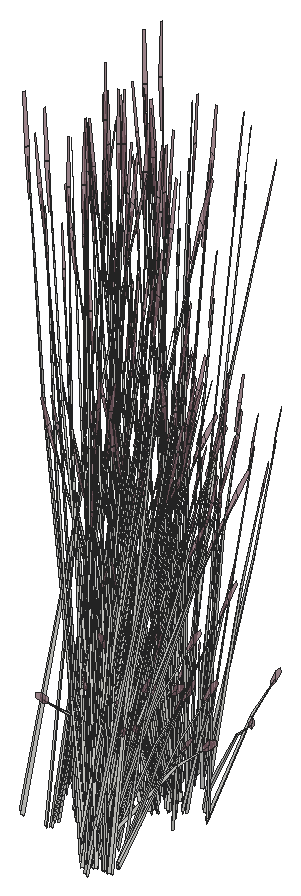
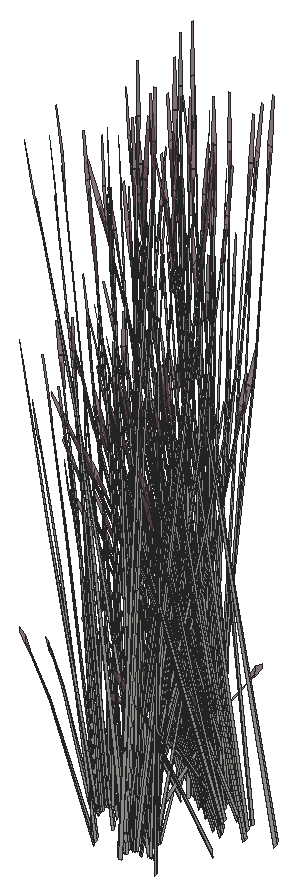
# SketchUp Ruby script. Lengths in inches.
U = 1.inch
M = Sketchup.active_model
def pt(a) = Geom::Point3d.new(a.map { |v| v * U })
def face(e, loops, mat)
  f = e.add_face(loops[0].map { |a| pt(a) })
  loops[1..].each { |l| e.add_face(l.map { |a| pt(a) }).erase! }
  f.material = f.back_material = mat if mat
  f
end
# faces: each face lists its corners as indices into pts; further lists are holes
def faces(e, pts, list, mat = nil) = list.each { |f| face(e, (f[0].is_a?(Array) ? f : [f]).map { |l| l.map { |i| pts[i] } }, mat) }
# xy, xz, yz: faces in a plane at the given z, y or x. An outline is a flat list of corners, or four numbers for a rectangle; further outlines are holes
def ring(l) = l.size == 4 ? [[l[0], l[1]], [l[2], l[1]], [l[2], l[3]], [l[0], l[3]]] : l.each_slice(2).to_a
def flat(e, list, mat, &to3) = list.each { |f| face(e, (f[0].is_a?(Array) ? f : [f]).map { |l| ring(l).map { |u, v| to3.(u, v) } }, mat) }
def xy(e, z, list, mat = nil) = flat(e, list, mat) { |x, y| [x, y, z] }
def xz(e, y, list, mat = nil) = flat(e, list, mat) { |x, z| [x, y, z] }
def yz(e, x, list, mat = nil) = flat(e, list, mat) { |y, z| [x, y, z] }
def lines(e, pts, list) = list.each { |a, b| e.add_line(pt(pts[a]), pt(pts[b])) }
# prism: a flat outline (further loops are holes) pulled along v
def prism(e, loops, v, mat = nil)
  f = face(e, loops, mat); d = Geom::Vector3d.new(v.map { |x| x * U })
  f.pushpull(f.normal.samedirection?(d) ? d.length : -d.length)
end
def box(e, o, s, mat = nil) = prism(e, [[o, [o[0] + s[0], o[1], o[2]], [o[0] + s[0], o[1] + s[1], o[2]], [o[0], o[1] + s[1], o[2]]]], [0, 0, s[2]], mat)
def at(x, y, z, deg = 0) = Geom::Transformation.translation(pt([x, y, z])) * Geom::Transformation.rotation(ORIGIN, Z_AXIS, deg.degrees)
def axes(o, x, y, z) = Geom::Transformation.new([*x, 0, *y, 0, *z, 0, *pt(o).to_a, 1])
def part(name) = M.definitions.add(name)
# library, detail: a bought-in or finely detailed component or shape, given as its bounding box
def library(name, o, s) = part(name).tap { |d| box(d.entities, o, s) }
def detail(e, o, s) = box(e.add_group.entities, o, s)
def put(e, d, t, mat = nil) = e.add_instance(d, t).tap { |i| i.material = mat if mat }
def group(e, t, mat = nil) = e.add_group.tap { |g| g.transformation = t; g.material = mat if mat }.entities
root = M.entities
M.materials.add("LightPink_Translucent").color = [144, 107, 117]
M.materials["LightPink_Translucent"].alpha = 0.75
c1 = part("blade")
p = [[2.15,0.21,22],[0,0.17,0],[0.09,0.45,0],[2.18,0.31,22],[2.29,0.31,22],[0.38,0.45,0],
  [2.48,0.24,33],[2.49,0.24,33],[2.48,0.22,33]]
faces(c1.entities,p,[[0,1,2,3],[4,5,2,3],[6,3,4,7],[8,0,3,6]])
c2 = part("seeds")
p = [[0.3,-0.1,1.38],[-0.01,-0.03,1.59],[-0.01,-0.03,0.03],[0.14,-0.07,-0.07],[0.29,-0.03,3],[0.15,0.01,3.11]]
faces(c2.entities,p,[[0,1,2,3],[1,0,4,5]],"LightPink_Translucent")
c3 = part("blade with seeds")
put(c3.entities,c1,at(0,0,0))
put(c3.entities,c2,axes([2.4,0.25,30.99],[1.5799,-0.05474,1.17369],[-0.12525,1.92788,0.29478],[-0.07173,-0.02425,1.56792]))
put(root,c3,axes([411.76,30.21,-9.7],[-0.40181,-0.39593,0.16428],[0.40492,-0.38402,0.32672],[-0.04438,0.08086,1.49371]))
put(root,c3,axes([411.01,29.61,-10.08],[0.53199,0.08911,-0.58063],[-0.11226,0.54969,-0.15239],[0.15876,0.06661,1.28164]))
put(root,c3,axes([413.37,30.57,-9.42],[-0.31598,0.08973,1.06958],[0.14873,-0.37085,0.78586],[0.16763,0.02538,0.23558]))
put(root,c3,axes([409.99,31.64,-9.95],[-0.51557,-0.24403,0],[0.24813,-0.50705,0],[0,0,1.51513]))
put(root,c3,axes([410.41,31,-9.7],[-0.49938,-0.43748,-0.23459],[0.42021,-0.49126,0.51337],[-0.13447,0.05118,1.56642]))
put(root,c3,axes([409.1,31.83,-9.69],[0.47863,0.27177,0.46235],[-0.28609,0.48733,0],[-0.10901,-0.0619,1.46668]))
put(root,c3,axes([405.94,33.55,-9.59],[-0.1827,-0.0161,1.33163],[-0.18717,-0.43188,-0.28638],[0.22444,-0.12218,0.56934]))
put(root,c3,axes([406.94,33.97,-7.62],[-0.0668,-0.00413,1.65179],[-0.27738,-0.44233,-0.15608],[0.11139,-0.14544,0.29231]))
put(root,c3,axes([410.79,29.95,-9.47],[0.24813,-0.48978,0.41661],[0.51557,0.23571,-0.2005],[0,0.1129,1.33761]))
put(root,c3,axes([413.22,32.14,-7.62],[-0.04624,-0.04758,1.65179],[0.10116,-0.51007,-0.15608],[0.18215,-0.03259,0.29231]))
put(root,c3,axes([406.15,32.76,-9.42],[-0.17034,0.27669,1.06958],[-0.14642,-0.37174,0.78586],[0.14069,-0.09315,0.23558]))
put(root,c3,axes([410.69,30.23,-9.87],[0,0.62861,-0.05249],[-0.63949,0,0],[0,0.01975,1.67027]))
put(root,c3,axes([410.74,29.79,-9.94],[0.30722,0.45622,-0.41661],[-0.46535,0.32126,0.2005],[0.09942,0.05645,1.33761]))
put(root,c3,axes([412.82,31.72,-8.34],[-0.09788,-0.45691,-0.03251],[0.46264,-0.10504,-0.14742],[0.09661,0.02897,0.48626]))
put(root,c3,axes([411.62,31.7,-7.3125],[0.02738,-0.55277,-0.11324],[0.51847,0.01511,-0.62851],[0.19968,0.0384,0.95501]))
put(root,c3,axes([405.91,33.8,-7.78],[0.44516,-0.07768,-0.32977],[0.11755,0.44407,0.42575],[0.12757,-0.11927,0.81462]))
put(root,c3,axes([412.09,30.23,-9.69],[0,-0.54355,0.46235],[0.57217,0,0],[0,0.1238,1.46668]))
put(root,c3,axes([410.66,30.63,-9.47],[0.55535,-0.03355,0.41661],[0.05022,0.55698,-0.2005],[-0.09942,0.05645,1.33761]))
put(root,c3,axes([411,30.06,-9.5625],[0.47648,-0.15851,0.13483],[0.16686,0.45265,-0.38503],[0,0.09962,1.18024]))
put(root,c3,axes([411.54,31.49,-7.3],[-0.29098,-0.34031,0.32977],[0.33226,-0.32215,-0.42575],[0.16881,0.04902,0.81462]))
put(root,c3,axes([410.16,30.9,-9.94],[-0.55535,0.03355,-0.41661],[-0.05022,-0.55698,0.2005],[-0.09942,0.05645,1.33761]))
put(root,c3,axes([412.77,31.17,-9.59],[-0.12317,-0.13368,1.33163],[0.16025,-0.44223,-0.28638],[0.24919,0.05991,0.56934]))
put(root,c3,axes([410.57,31.65,-9.95],[0.51557,0.24403,0],[-0.24813,0.50705,0],[0,0,1.62917]))
put(root,c3,axes([412.07,31.37,-7.61],[0.10971,-0.00919,1.62908],[0.30091,-0.42228,-0.25764],[0.19514,0.05574,0.13065]))
put(root,c3,axes([410.78,32.19,-9.96],[-0.31576,-0.54657,-0.04789],[0.53494,-0.30375,0.48057],[-0.13182,0.05204,1.52373]))
put(root,c3,axes([410.67,30.87,-9.5625],[0.37783,0.32657,0.13483],[-0.31516,0.36844,-0.38503],[-0.08772,0.04981,1.18024]))
put(root,c3,axes([405.95,33.99,-7.6],[0.35109,0.22859,0.05988],[-0.2044,0.32553,0.47138],[0.11256,-0.10524,0.71878]))
put(root,c3,axes([405.85,33.9,-7.59],[0.12683,0.50025,0.447],[-0.49754,0.08682,0.36857],[0.14663,-0.11765,0.92496]))
put(root,c3,axes([407.19,34.5,-7.61],[0.07097,-0.08279,1.62908],[-0.09083,-0.50786,-0.25764],[0.17806,-0.09629,0.13065]))
put(root,c3,axes([411.64,31.4375,-7.36],[0.51122,0.01309,-0.66157],[-0.03434,0.5511,0.07984],[0.21658,0.05816,0.93586]))
put(root,c3,axes([411.07,31.88,-9.69],[0.47863,-0.27177,0.46235],[0.28609,0.48733,0],[-0.10901,0.0619,1.46668]))
put(root,c3,axes([410.39,31.45,-9.87],[0.22235,0.62444,-0.05599],[-0.63531,0.21881,0],[0.00776,0.02181,1.60327]))
put(root,c3,axes([410.63,32.125,-10.11],[-0.47712,-0.13449,-0.28847],[0.12013,-0.47362,0.28847],[-0.09619,0.05462,1.29413]))
put(root,c3,axes([412.48,30.32,-9.79],[0.63949,0,0],[0,0.60749,-0.48057],[0,0.13836,1.52448]))
put(root,c3,axes([412.22,30.63,-9.95],[-0.63917,-0.00435,-0.04634],[0,-0.60749,0.46507],[-0.02009,0.13829,1.47457]))
put(root,c3,axes([410.84,30.1,-9.52],[0.57594,0.25935,-0.27094],[-0.27732,0.5474,-0.46562],[0.0181,0.1344,1.4872]))
put(root,c3,axes([411.95,31.66,-7.78],[0.29098,0.34031,-0.32977],[-0.33226,0.32215,0.42575],[0.16881,0.04902,0.81462]))
put(root,c3,axes([412.09,30.72,-10.11],[-0.35699,0.33913,-0.28847],[-0.35699,-0.33913,0.28847],[0,0.10923,1.29413]))
put(root,c3,axes([410.55,30.75,-9.52],[0.05959,0.62022,-0.27094],[-0.62068,0.0375,-0.46562],[-0.1093,0.08261,1.4872]))
put(root,c3,axes([411.8,31.79,-7.6],[-0.02575,0.41332,0.05988],[-0.38885,-0.01133,0.47138],[0.14895,0.04325,0.71878]))
put(root,c3,axes([410.78,30.51,-9.94],[-0.24813,0.48978,-0.41661],[-0.51557,-0.23571,0.2005],[0,0.1129,1.33761]))
put(root,c3,axes([411.84,31.66,-7.59],[-0.37709,0.35815,0.447],[-0.32522,-0.38035,0.36857],[0.17692,0.06607,0.92496]))
put(root,c3,axes([405.79,35.27,-7.3125],[-0.25732,-0.49218,-0.11324],[0.45669,-0.24187,-0.62851],[0.19245,-0.06494,0.95501]))
put(root,c3,axes([405.77,34.85,-7.64],[0.13855,-0.49442,-0.47583],[0.47502,0.16947,-0.36857],[0.19125,-0.04534,0.91046]))
put(root,c3,axes([405.02,32.84,-9.79],[0.31974,-0.54466,0],[0.53494,0.30375,-0.48057],[0.12184,0.06918,1.52448]))
put(root,c3,axes([406.28,34.99,-10.15],[-0.32938,0.06523,1.31842],[-0.05243,-0.51922,0.07547],[0.2307,-0.07859,0.75023]))
put(root,c3,axes([406.88,34.53,-9.89],[-0.31706,-0.34757,-0.06041],[0.34725,-0.31847,-0.27392],[0.09839,-0.02242,0.90349]))
put(root,c3,axes([410.64,32.08,-7.3],[-0.07899,-0.43781,0.32977],[0.45153,-0.11561,-0.42575],[0.12128,0.12546,0.81462]))
put(root,c3,axes([410.79,31.91,-9.83],[0.64025,0.17667,0.2864],[-0.16018,0.63149,-0.33981],[-0.10597,0.07904,1.53541]))
put(root,c3,axes([410.74,32.34,-10.12],[-0.47863,0.27177,-0.46235],[-0.28609,-0.48733,0],[-0.10901,0.0619,1.46668]))
put(root,c3,axes([412.33,30.73,-10.12],[0,0.54355,-0.46235],[-0.57217,0,0],[0,0.1238,1.46668]))
put(root,c3,axes([405.68,35.03,-7.36],[0.44939,-0.24006,-0.66157],[0.25044,0.49415,0.07984],[0.21713,-0.05613,0.93586]))
put(root,c3,axes([410.9,30.79,-8.39],[-0.18996,-0.09365,1.59586],[0.39312,-0.39287,0.12904],[0.24502,0.17723,0.68222]))
put(root,c3,axes([410.94,29.56,-7.83],[-0.44191,-0.28242,1.28769],[0.46662,-0.43971,0.5556],[0.14258,0.26499,1.24467]))
put(root,c3,axes([411.61,31.86,-9.42],[-0.28795,-0.15629,1.06958],[0.37181,-0.1588,0.78586],[0.10029,0.13452,0.23558]))
put(root,c3,axes([410.6,32.3,-7.3125],[0.30474,-0.46525,-0.11324],[0.44133,0.26804,-0.62851],[0.15341,0.13145,0.95501]))
put(root,c3,axes([405.62,35.125,-7.3],[-0.42502,-0.15163,0.32977],[0.12396,-0.44238,-0.42575],[0.17112,-0.04056,0.81462]))
put(root,c3,axes([402.71,33.8,-10.52],[-0.50338,0.21762,1.20058],[-0.16022,-0.62439,0.4665],[0.30911,0.01039,1.36553]))
put(root,c3,axes([409.25,37.59,-7.61],[-0.07822,-0.07621,1.62908],[-0.52201,0.04832,-0.25764],[-0.08331,-0.18228,0.13065]))
put(root,c3,axes([410.46,38.49,-9.59],[-0.14537,0.11002,1.33163],[-0.43536,-0.19256,-0.28638],[0.0807,-0.23948,0.56934]))
put(root,c3,axes([406.64,34.65,-10.61],[-0.02673,-0.08252,1.6421],[0.18538,-0.48271,-0.25086],[0.187,-0.00694,0.2797]))
put(root,c3,axes([409.8,38.875,-7.36],[-0.24409,-0.44196,-0.66157],[0.50245,-0.2463,0.07984],[-0.05708,-0.21354,0.93586]))
put(root,c3,axes([408.59,31.68,-7.3],[0.34603,-0.28618,0.32977],[0.32756,0.32677,-0.42575],[-0.04984,0.16603,0.81462]))
put(root,c3,axes([411.18,32.26,-9.79],[0.31974,0.54466,0],[-0.53494,0.30375,-0.48057],[-0.12184,0.06918,1.52448]))
put(root,c3,axes([410.2,32.69,-7.62],[0.00151,-0.06581,1.65179],[0.43826,-0.29033,-0.15608],[0.15223,0.10363,0.29231]))
put(root,c3,axes([411.6875,32.4375,-10.61],[0.03726,-0.07847,1.6421],[0.46909,-0.23111,-0.25086],[0.14221,0.11962,0.2797]))
put(root,c3,axes([410.91,30.1,-9.35],[-0.01397,-0.51177,1.31553],[0.63227,0.13266,0.557],[-0.14954,0.28003,1.24175]))
put(root,c3,axes([411.07,30.66,-10.05],[0.18752,0.49766,-0.6445],[-0.54017,0.17923,-0.16915],[0.02073,0.16852,1.42262]))
put(root,c3,axes([410.96,32.07,-7.64],[0.50465,-0.12921,-0.47583],[0.08828,0.48932,-0.36857],[0.13555,0.14022,0.91046]))
put(root,c3,axes([409.38,37.9,-10.61],[-0.08578,0.01958,1.6421],[-0.47437,-0.22044,-0.25086],[0.00796,-0.18387,0.2797]))
put(root,c3,axes([409.56,32.15,-7.3],[0.15418,-0.41799,0.32977],[0.44981,0.12192,-0.42575],[0.04124,0.16829,0.81462]))
put(root,c3,axes([406.0625,35.08,-7.78],[0.42502,0.15163,-0.32977],[-0.12396,0.44238,0.42575],[0.17112,-0.04056,0.81462]))
put(root,c3,axes([410.82,39.31,-7.36],[0.01331,-0.50278,-0.66157],[0.56035,0.03377,0.07984],[0.05914,-0.213,0.93586]))
put(root,c3,axes([405.3125,33.17,-10.12],[0.47863,0.27177,-0.46235],[-0.28609,0.48733,0],[0.10901,0.0619,1.46668]))
put(root,c3,axes([411.65,32.57,-9.52],[-0.32795,-0.01705,0.97832],[0.21658,-0.36206,0.54015],[0.12956,0.12863,0.76741]))
put(root,c3,axes([411.6,38.52,-7.61],[-0.00494,-0.10818,1.62908],[-0.41695,-0.31265,-0.25764],[0.06446,-0.18952,0.13065]))
put(root,c3,axes([409.85,38.5,-7.78],[0.15418,-0.41799,-0.32977],[0.44981,0.12192,0.42575],[-0.04124,-0.16829,0.81462]))
put(root,c3,axes([410.1875,39.05,-8.39],[-0.09522,0.18683,1.59586],[-0.39947,-0.38663,0.12904],[0.18021,-0.24097,0.68222]))
put(root,c3,axes([411.49,38.13,-7.62],[-0.05194,0.04152,1.65179],[-0.50886,-0.14007,-0.15608],[-0.01842,-0.18118,0.29231]))
put(root,c3,axes([410.71,32.47,-7.6],[-0.23243,0.34529,0.05988],[-0.331,-0.20103,0.47138],[0.10701,0.1107,0.71878]))
put(root,c3,axes([410.16,33.64,-6.74],[0.35341,-0.31182,-0.06041],[0.32382,0.34152,-0.27392],[0.0228,0.09677,0.90349]))
put(root,c3,axes([404.9,34.53,-8.39],[-0.21212,0.01231,1.59586],[0.14072,-0.53355,0.12904],[0.3023,0.033,0.68222]))
put(root,c3,axes([410.81,32.38,-7.59],[-0.50866,0.12474,0.447],[-0.08828,-0.48932,0.36857],[0.11963,0.14421,0.92496]))
put(root,c3,axes([409.62,38.79,-7.64],[-0.50273,-0.13626,-0.47583],[0.17232,-0.46717,-0.36857],[-0.0461,-0.18809,0.91046]))
put(root,c3,axes([409.93,37.62,-9.42],[0.06561,0.31695,1.06958],[-0.36394,-0.17555,0.78586],[0.03916,-0.16229,0.23558]))
put(root,c3,axes([406,35.26,-7.6],[0.18783,0.37061,0.05988],[-0.34252,0.1814,0.47138],[0.15099,-0.03579,0.71878]))
put(root,c3,axes([410.7,39.14,-7.64],[-0.3661,-0.36521,-0.47583],[0.38674,-0.31985,-0.36857],[0.0557,-0.18556,0.91046]))
put(root,c3,axes([405.96,35.13,-7.59],[-0.14449,0.4956,0.447],[-0.47502,-0.16947,0.36857],[0.1868,-0.02978,0.92496]))
put(root,c3,axes([410.58,31.69,-9.59],[0.00902,-0.18018,1.33163],[0.43127,-0.20126,-0.28638],[0.13313,0.21566,0.56934]))
put(root,c3,axes([409.42,32.53,-7.6],[-0.37684,0.18473,0.05988],[-0.18445,-0.33686,0.47138],[0.03639,0.14849,0.71878]))
put(root,c3,axes([408.37,31.75,-6.97],[0.56206,0.02693,-0.12569],[-0.01536,0.50991,-0.69765],[-0.03904,0.19638,1.06006]))
put(root,c3,axes([409.41,32.32,-7.3125],[0.50045,-0.25306,-0.11324],[0.24593,0.44915,-0.62851],[0.06603,0.18927,0.95501]))
put(root,c3,axes([409.55,32.49,-7.28],[-0.50393,-0.1421,0.49617],[0.17232,-0.46717,0.40911],[0.03028,0.18372,1.0267]))
put(root,c3,axes([408.63,33.19,-9.42],[-0.01324,-0.32319,1.06958],[0.33072,0.23052,0.78586],[-0.06504,0.15405,0.23558]))
put(root,c3,axes([409.9,38.6,-7.59],[0.50393,0.1421,0.447],[-0.17232,0.46717,0.36857],[-0.03028,-0.18372,0.92496]))
put(root,c3,axes([410.05,38.76,-7.3125],[-0.50045,0.25306,-0.11324],[-0.24593,-0.44915,-0.62851],[-0.06603,-0.18927,0.95501]))
put(root,c3,axes([411.09,39.33,-7.3125],[-0.56206,-0.02693,-0.11324],[0.01536,-0.50991,-0.62851],[0.03904,-0.19638,0.95501]))
put(root,c3,axes([404.61,34.21,-10.08],[0.53199,0.08911,-0.58063],[-0.11226,0.54969,-0.15239],[0.15876,0.06661,1.28164]))
put(root,c3,axes([411.05,39.01,-7.78],[0.34603,-0.28618,-0.32977],[0.32756,0.32677,0.42575],[0.04984,-0.16603,0.81462]))
put(root,c3,axes([410.04,38.5625,-7.6],[0.37684,-0.18473,0.05988],[0.18445,0.33686,0.47138],[-0.03639,-0.14849,0.71878]))
put(root,c3,axes([406.96,35.17,-9.42],[-0.31598,0.08973,1.06958],[0.14873,-0.37085,0.78586],[0.16763,0.02538,0.23558]))
put(root,c3,axes([409.5,32.42,-10.61],[0.08277,-0.02958,1.6421],[0.49786,0.16279,-0.25086],[0.01456,0.18348,0.2797]))
put(root,c3,axes([408.75,31.95,-7.34],[0.3661,0.36521,-0.52818],[-0.38674,0.31985,-0.40911],[-0.0557,0.18556,1.01061]))
put(root,c3,axes([406.82,36.74,-7.62],[-0.04624,-0.04758,1.65179],[0.10116,-0.51007,-0.15608],[0.18215,-0.03259,0.29231]))
put(root,c3,axes([408.35,32.5,-9.37],[0.46459,-0.09625,0.0606],[0.10681,0.38778,-0.80367],[-0.02945,0.1963,0.72038]))
put(root,c3,axes([409.84,32.3,-7.64],[0.50273,0.13626,-0.47583],[-0.17232,0.46717,-0.36857],[0.0461,0.18809,0.91046]))
put(root,c3,axes([410.12,31.34,-8.39],[-0.1169,-0.17452,1.59586],[0.54019,-0.14692,0.12904],[0.12209,0.27397,0.68222]))
put(root,c3,axes([406.42,36.31,-8.34],[-0.09788,-0.45691,-0.03251],[0.46264,-0.10504,-0.14742],[0.09661,0.02897,0.48626]))
put(root,c3,axes([405.22,36.3,-7.3125],[0.02738,-0.55277,-0.11324],[0.51847,0.01511,-0.62851],[0.19968,0.0384,0.95501]))
put(root,c3,axes([409.61,32.59,-7.78],[-0.15418,0.41799,-0.32977],[-0.44981,-0.12192,0.42575],[0.04124,0.16829,0.81462]))
put(root,c3,axes([408.67,40.54,-10.05],[-0.21003,-0.55738,-0.65031],[0.60499,-0.20074,-0.17068],[-0.02321,-0.18874,1.43544]))
put(root,c3,axes([411.48,38.83,-10.61],[-0.07655,-0.04282,1.6421],[-0.19662,-0.47839,-0.25086],[0.13264,-0.12982,0.2797]))
put(root,c3,axes([408.64,31.78,-7.03],[-0.01331,0.50278,-0.73435],[-0.56035,-0.03377,0.08862],[-0.05914,0.213,1.03881]))
put(root,c3,axes([405.14,36.08,-7.3],[-0.29098,-0.34031,0.32977],[0.33226,-0.32215,-0.42575],[0.16881,0.04902,0.81462]))
put(root,c3,axes([409.9,38.94,-7.3],[-0.15418,0.41799,0.32977],[-0.44981,-0.12192,-0.42575],[-0.04124,-0.16829,0.81462]))
put(root,c3,axes([409.17,31.42,-8.39],[-0.01252,-0.20862,1.59586],[0.54251,0.1384,0.12904],[-0.03356,0.2973,0.68222]))
put(root,c3,axes([406.37,35.76,-9.59],[-0.12317,-0.13368,1.33163],[0.16025,-0.44223,-0.28638],[0.24919,0.05991,0.56934]))
put(root,c3,axes([411.05,39.12,-7.59],[0.36417,0.37086,0.447],[-0.38674,0.31985,0.36857],[0.06718,-0.174,0.92496]))
put(root,c3,axes([411.18,39.15,-7.6],[0.42027,0.02533,0.05988],[-0.01152,0.38243,0.47138],[0.04398,-0.14649,0.71878]))
put(root,c3,axes([410.87,39.41,-7.3],[-0.34603,0.28618,0.32977],[-0.32756,-0.32677,-0.42575],[0.04984,-0.16603,0.81462]))
put(root,c3,axes([409.65,32.21,-7.36],[0.24409,0.44196,-0.66157],[-0.50245,0.2463,0.07984],[0.05708,0.21354,0.93586]))
put(root,c3,axes([411.48,40.18,-7.36],[0.26714,-0.42887,-0.66157],[0.46811,0.30479,0.07984],[0.1595,-0.15539,0.93586]))
put(root,c3,axes([408.59,38.93,-9.79],[-0.31974,-0.54466,0],[0.53494,-0.30375,-0.48057],[0.12184,-0.06918,1.52448]))
put(root,c3,axes([411.47,39.98,-7.64],[-0.13138,-0.49631,-0.47583],[0.49754,-0.08682,-0.36857],[0.14258,-0.13331,0.91046]))
put(root,c3,axes([405.67,35.96,-7.61],[0.10971,-0.00919,1.62908],[0.30091,-0.42228,-0.25764],[0.19514,0.05574,0.13065]))
put(root,c3,axes([409.29,38.28,-10.02],[-0.35341,0.31182,-0.03625],[-0.32382,-0.34152,-0.16435],[-0.0228,-0.09677,0.54209]))
put(root,c3,axes([409.29,33.33,-7.61],[0.06483,0.08753,1.62908],[0.52315,0.03439,-0.25764],[0.05261,0.19303,0.13065]))
put(root,c3,axes([411.7,40.34,-7.3125],[-0.47307,-0.29971,-0.11324],[0.27254,-0.43404,-0.62851],[0.13365,-0.15087,0.95501]))
put(root,c3,axes([405.24,36.03,-7.36],[0.51122,0.01309,-0.66157],[-0.03434,0.5511,0.07984],[0.21658,0.05816,0.93586]))
put(root,c3,axes([407.44,40.46,-10.12],[0,-0.54355,-0.46235],[0.57217,0,0],[0,-0.1238,1.46668]))
put(root,c3,axes([409.02,38.85,-10.12],[0.47863,-0.27177,-0.46235],[0.28609,0.48733,0],[0.10901,-0.0619,1.46668]))
put(root,c3,axes([411.87,39.79,-9.59],[-0.1827,-0.0161,1.33163],[-0.18717,-0.43188,-0.28638],[0.22444,-0.12218,0.56934]))
put(root,c3,axes([412.86,40.21,-7.62],[-0.0668,-0.00413,1.65179],[-0.27738,-0.44233,-0.15608],[0.11139,-0.14544,0.29231]))
put(root,c3,axes([408.45,32.49,-8.87],[0.01124,-0.2806,1.43727],[0.50537,0.14821,0.19862],[-0.04379,0.29905,0.67868]))
put(root,c3,axes([409.59,39.96,-10.08],[0.34446,-0.40855,-0.58063],[0.42791,0.37046,-0.15239],[0.13803,-0.10191,1.28164]))
put(root,c3,axes([412.08,38.99,-9.42],[-0.17034,0.27669,1.06958],[-0.14642,-0.37174,0.78586],[0.14069,-0.09315,0.23558]))
put(root,c3,axes([405.55,36.26,-7.78],[0.29098,0.34031,-0.32977],[-0.33226,0.32215,0.42575],[0.16881,0.04902,0.81462]))
put(root,c3,axes([405.4,36.39,-7.6],[-0.02575,0.41332,0.05988],[-0.38885,-0.01133,0.47138],[0.14895,0.04325,0.71878]))
put(root,c3,axes([411.83,40.03,-7.78],[0.44516,-0.07768,-0.32977],[0.11755,0.44407,0.42575],[0.12757,-0.11927,0.81462]))
put(root,c3,axes([405.4375,36.26,-7.59],[-0.37709,0.35815,0.447],[-0.32522,-0.38035,0.36857],[0.17692,0.06607,0.92496]))
put(root,c3,axes([408.99,40.68,-9.94],[0.24813,-0.48978,-0.41661],[0.51557,0.23571,0.2005],[0,-0.1129,1.33761]))
put(root,c3,axes([409.22,40.4375,-9.52],[-0.05959,-0.62022,-0.27094],[0.62068,-0.0375,-0.46562],[0.1093,-0.08261,1.4872]))
put(root,c3,axes([407.68,40.47,-10.11],[0.35699,-0.33913,-0.28847],[0.35699,0.33913,0.28847],[0,-0.10923,1.29413]))
put(root,c3,axes([411.47,40.3,-7.3],[-0.44516,0.07768,0.32977],[-0.11755,-0.44407,-0.42575],[0.12757,-0.11927,0.81462]))
put(root,c3,axes([408.93,41.09,-9.52],[-0.57594,-0.25935,-0.27094],[0.27732,-0.5474,-0.46562],[-0.0181,-0.1344,1.4872]))
put(root,c3,axes([409.14,39.0625,-10.11],[0.47712,0.13449,-0.28847],[-0.12013,0.47362,0.28847],[0.09619,-0.05462,1.29413]))
put(root,c3,axes([404.5,35.38,-8.39],[-0.18996,-0.09365,1.59586],[0.39312,-0.39287,0.12904],[0.24502,0.17723,0.68222]))
put(root,c3,axes([404.2,36.9,-7.3125],[0.30474,-0.46525,-0.11324],[0.44133,0.26804,-0.62851],[0.15341,0.13145,0.95501]))
put(root,c3,axes([411.87,40.23,-7.6],[0.35109,0.22859,0.05988],[-0.2044,0.32553,0.47138],[0.11256,-0.10524,0.71878]))
put(root,c3,axes([411.77,40.13,-7.59],[0.12683,0.50025,0.447],[-0.49754,0.08682,0.36857],[0.14663,-0.11765,0.92496]))
put(root,c3,axes([413.12,40.73,-7.61],[0.07097,-0.08279,1.62908],[-0.09083,-0.50786,-0.25764],[0.17806,-0.09629,0.13065]))
put(root,c3,axes([405.29,37.03,-10.61],[0.03726,-0.07847,1.6421],[0.46909,-0.23111,-0.25086],[0.14221,0.11962,0.2797]))
put(root,c3,axes([404.56,36.67,-7.64],[0.50465,-0.12921,-0.47583],[0.08828,0.48932,-0.36857],[0.13555,0.14022,0.91046]))
put(root,c3,axes([409.3,40.92,-9.73],[0.57623,0.26344,0.22409],[-0.27732,0.5474,0.46562],[0,-0.12618,1.49497]))
put(root,c3,axes([409.08,41.66,-9.73],[0.13555,-0.64407,-0.21817],[0.64269,0.11227,0.47743],[-0.1123,-0.08895,1.45677]))
put(root,c3,axes([409.11,40.56,-9.47],[-0.55535,0.03355,0.41661],[-0.05022,-0.55698,-0.2005],[0.09942,-0.05645,1.33761]))
put(root,c3,axes([407.68,40.96,-9.69],[0,0.54355,0.46235],[-0.57217,0,0],[0,-0.1238,1.46668]))
put(root,c3,axes([411.72,41.51,-7.3125],[-0.25732,-0.49218,-0.11324],[0.45669,-0.24187,-0.62851],[0.19245,-0.06494,0.95501]))
put(root,c3,axes([411.7,41.08,-7.64],[0.13855,-0.49442,-0.47583],[0.47502,0.16947,-0.36857],[0.19125,-0.04534,0.91046]))
put(root,c3,axes([410.95,39.07,-9.79],[0.31974,-0.54466,0],[0.53494,0.30375,-0.48057],[0.12184,0.06918,1.52448]))
put(root,c3,axes([409.09,40.76,-9.8],[0.22235,0.6078,0.42607],[-0.63531,0.21135,0.16719],[0.00776,-0.11168,1.47927]))
put(root,c3,axes([412.2,41.22,-10.15],[-0.32938,0.06523,1.31842],[-0.05243,-0.51922,0.07547],[0.2307,-0.07859,0.75023]))
put(root,c3,axes([412.8,40.76,-9.89],[-0.31706,-0.34757,-0.06041],[0.34725,-0.31847,-0.27392],[0.09839,-0.02242,0.90349]))
put(root,c3,axes([408.98,41.24,-9.47],[-0.24813,0.48978,0.41661],[-0.51557,-0.23571,-0.2005],[0,-0.1129,1.33761]))
put(root,c3,axes([409.89,40.81,-9.95],[0,-0.62892,0],[0.63949,0,0],[0,0,1.6711]))
put(root,c3,axes([410.67,39.35,-9.69],[-0.47863,-0.27177,0.46235],[0.28609,-0.48733,0],[0.10901,0.0619,1.46668]))
put(root,c3,axes([411.61,41.26,-7.36],[0.44939,-0.24006,-0.66157],[0.25044,0.49415,0.07984],[0.21713,-0.05613,0.93586]))
put(root,c3,axes([409.59,40.41,-9.8],[-0.42403,0.49328,0.42607],[-0.50377,-0.43543,0.16719],[0.10223,-0.04923,1.47927]))
put(root,c3,axes([410.05,41.3,-9.86],[-0.47569,-0.46784,-0.05709],[0.47598,-0.46812,0],[-0.01661,-0.01634,1.63492]))
put(root,c3,axes([408.86,39.6,-9.7],[-0.14774,0.54019,0.16428],[-0.54062,-0.15287,0.32672],[0.09339,-0.00263,1.49371]))
put(root,c3,axes([411.54,41.36,-7.3],[-0.42502,-0.15163,0.32977],[0.12396,-0.44238,-0.42575],[0.17112,-0.04056,0.81462]))
put(root,c3,axes([408.63,40.04,-10.52],[-0.50338,0.21762,1.20058],[-0.16022,-0.62439,0.4665],[0.30911,0.01039,1.36553]))
put(root,c3,axes([409.98,40.2,-9.5625],[0.09866,-0.48509,0.13483],[0.48202,0.0842,-0.38503],[0.08772,0.04981,1.18024]))
put(root,c3,axes([404.29,44.68,-8.39],[-0.09522,0.18683,1.59586],[-0.39947,-0.38663,0.12904],[0.18021,-0.24097,0.68222]))
put(root,c3,axes([409.15,41.35,-9.8],[0.64638,0.11452,0.42607],[-0.13155,0.64678,0.16719],[-0.09446,-0.06245,1.47927]))
put(root,c3,axes([412.5625,40.88,-10.61],[-0.02673,-0.08252,1.6421],[0.18538,-0.48271,-0.25086],[0.187,-0.00694,0.2797]))
put(root,c3,axes([409.78,40.33,-9.47],[-0.30722,-0.45622,0.41661],[0.46535,-0.32126,-0.2005],[0.09942,0.05645,1.33761]))
put(root,c3,axes([408.8,42.39,-9.7],[0.54955,-0.14427,0.16428],[0.1357,0.53689,0.32672],[-0.04901,-0.07823,1.49371]))
put(root,c3,axes([409.94,40.36,-9.52],[0.51635,-0.36087,-0.27094],[0.34336,0.5099,-0.46562],[0.1274,0.05178,1.4872]))
